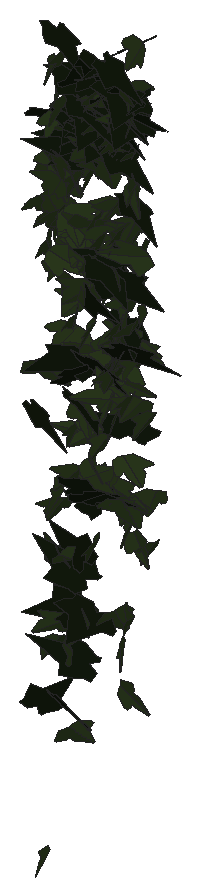
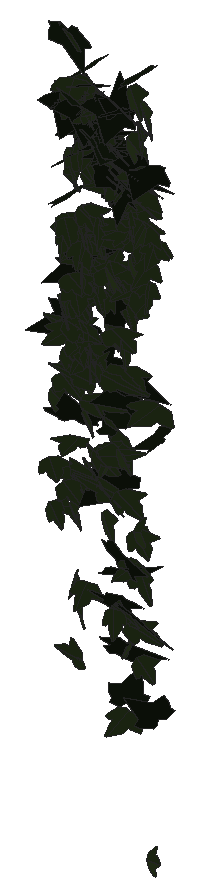
# SketchUp Ruby script. Lengths in millimetres.
U = 1.mm
M = Sketchup.active_model
def pt(a) = Geom::Point3d.new(a.map { |v| v * U })
def face(e, loops, mat)
  f = e.add_face(loops[0].map { |a| pt(a) })
  loops[1..].each { |l| e.add_face(l.map { |a| pt(a) }).erase! }
  f.material = f.back_material = mat if mat
  f
end
# faces: each face lists its corners as indices into pts; further lists are holes
def faces(e, pts, list, mat = nil) = list.each { |f| face(e, (f[0].is_a?(Array) ? f : [f]).map { |l| l.map { |i| pts[i] } }, mat) }
# xy, xz, yz: faces in a plane at the given z, y or x. An outline is a flat list of corners, or four numbers for a rectangle; further outlines are holes
def ring(l) = l.size == 4 ? [[l[0], l[1]], [l[2], l[1]], [l[2], l[3]], [l[0], l[3]]] : l.each_slice(2).to_a
def flat(e, list, mat, &to3) = list.each { |f| face(e, (f[0].is_a?(Array) ? f : [f]).map { |l| ring(l).map { |u, v| to3.(u, v) } }, mat) }
def xy(e, z, list, mat = nil) = flat(e, list, mat) { |x, y| [x, y, z] }
def xz(e, y, list, mat = nil) = flat(e, list, mat) { |x, z| [x, y, z] }
def yz(e, x, list, mat = nil) = flat(e, list, mat) { |y, z| [x, y, z] }
def lines(e, pts, list) = list.each { |a, b| e.add_line(pt(pts[a]), pt(pts[b])) }
# prism: a flat outline (further loops are holes) pulled along v
def prism(e, loops, v, mat = nil)
  f = face(e, loops, mat); d = Geom::Vector3d.new(v.map { |x| x * U })
  f.pushpull(f.normal.samedirection?(d) ? d.length : -d.length)
end
def box(e, o, s, mat = nil) = prism(e, [[o, [o[0] + s[0], o[1], o[2]], [o[0] + s[0], o[1] + s[1], o[2]], [o[0], o[1] + s[1], o[2]]]], [0, 0, s[2]], mat)
def at(x, y, z, deg = 0) = Geom::Transformation.translation(pt([x, y, z])) * Geom::Transformation.rotation(ORIGIN, Z_AXIS, deg.degrees)
def axes(o, x, y, z) = Geom::Transformation.new([*x, 0, *y, 0, *z, 0, *pt(o).to_a, 1])
def part(name) = M.definitions.add(name)
# library, detail: a bought-in or finely detailed component or shape, given as its bounding box
def library(name, o, s) = part(name).tap { |d| box(d.entities, o, s) }
def detail(e, o, s) = box(e.add_group.entities, o, s)
def put(e, d, t, mat = nil) = e.add_instance(d, t).tap { |i| i.material = mat if mat }
def group(e, t, mat = nil) = e.add_group.tap { |g| g.transformation = t; g.material = mat if mat }.entities
root = M.entities
M.materials.add("efeu1").color = [18, 25, 13]
M.materials.add("efeu2").color = [43, 57, 29]
c1 = part("ivyleaf_10")
p = [[0,12.8,-0.8],[-1.5,51.3,-10.9],[-4.9,51,-11.6],[-13.6,26.5,-7.3],[-13.2,15.9,-4.6],[-21.1,19.3,-7.2],
  [-29.5,16.3,-8.3],[-29.2,8.3,-6.2],[-19.7,-9.8,0.5],[-7.6,-13,4],[1,-12.2,5.8],[-0.4,51.1,-11.1],
  [-1.5,51.1,-10.9],[1,-12.4,5.9],[16.9,-12.4,3.5],[35.1,9.1,-5.1],[35,12.9,-6.1],[20.5,16.4,-4.9],
  [15.8,15,-3.8],[15.3,27.6,-7.1],[12.8,31.3,-7.8]]
faces(c1.entities,p,[[0,1,2,3,4,5,6,7,8,9,10],[11,12,0,13,14,15,16,17,18,19,20]],"efeu2")
c2 = part("ivyleaf_9")
p = [[39.1,54.8,31.7],[34.5,51.8,30.2],[-5.3,25.2,17.3],[-17.9,28.3,20.9],[-21.6,21.7,17],[-20.2,4.3,5.3],
  [-22.9,-0.3,2.5],[-17.1,-4,-0.6],[-2,-2.1,-1.2],[-0.7,-15.4,-10.1],[16.6,-22.3,-16.7],[21.1,-15.1,-12.5],
  [32.7,-10.7,-11],[46.1,-1.8,-6.6],[30.8,11.2,3.8]]
faces(c2.entities,p,[[0,1,2,3,4,5,6,7,8,9,10,11,12,13,14]],"efeu1")
put(root,c1,axes([1082.1,997.6,1167.9],[-0.50064,-0.61,-0.35285],[0.27301,0.3224,-0.66429],[1.31311,-0.2996,0.00358]))
put(root,c1,axes([1101.4,1010.7,594.9],[-0.91283,0.27362,0.57924],[-0.97949,0.2663,-0.55195],[-0.726,-0.70331,0.01636]))
put(root,c1,axes([1078.7,1010.7,105.8],[0.19332,-0.35249,0.55094],[0.37543,-0.51507,-0.36591],[1.18682,0.22035,0.02601]))
put(root,c1,axes([1074.1,1009.7,891.8],[-1.05756,-0.30294,-0.44533],[0.73832,0.21874,-0.63287],[0.71108,-0.67767,-0.0052]))
put(root,c1,axes([1088.7,1021.1,449.9],[-0.25395,-0.6181,0.25042],[-0.05666,-0.24961,-0.63195],[1.26798,-0.13495,0.02191]))
put(root,c1,axes([1084.8,1003.8,1095.4],[0.04007,-0.60352,-0.39627],[0.15482,0.3959,-0.59863],[1.36534,-0.02718,0.07951]))
put(root,c1,axes([1092.3,1026.2,670.5],[-0.45383,-0.63166,0.16282],[-0.10698,-0.15281,-0.67517],[1.23686,-0.24499,0.00134]))
put(root,c1,axes([1082.9,1012,1137.2],[-0.40105,-0.48424,-0.52608],[0.41583,0.47861,-0.52806],[1.29573,-0.30348,0.00664]))
put(root,c2,axes([1076.6,999.2,351.1],[-0.19601,-0.125,0.77139],[1.22033,0.43123,0.15549],[-0.85013,0.64784,0.04534]))
put(root,c2,axes([1089.8,1004.8,1306.5],[0.94112,0.57643,-0.03673],[-0.03109,-0.03438,-0.7594],[-1.09884,0.49466,-0.00998]))
put(root,c1,axes([1088.6,1027.2,680.6],[0.18777,-0.34057,0.59703],[0.34191,-0.56941,-0.3545],[1.26267,0.20483,0.00721]))
put(root,c1,axes([1088.2,1014.1,1202.2],[-1.29311,0.17274,-0.25591],[0.38946,-0.21125,-0.6859],[-0.44002,-0.69462,0.14496]))
put(root,c1,axes([1093.1,1017.7,1201.6],[-0.82238,0.6065,-0.06494],[-0.00615,-0.08186,-0.74301],[-1.16087,-0.42922,0.04994]))
put(root,c2,axes([1078,986.1,831.8],[0.78555,-0.62654,-0.12931],[-0.11182,0.11611,-0.75014],[1.21242,0.41666,0.0146]))
put(root,c1,axes([1094.3,1004.2,1165.7],[-0.99959,-0.46966,-0.21119],[0.33178,0.12169,-0.70416],[0.92221,-0.55285,0.02442]))
put(root,c1,axes([1100.8,1014.2,1059.6],[-0.24643,-0.28298,-0.65862],[-0.37765,-0.62898,0.30926],[-1.31099,0.23438,0.03472]))
put(root,c1,axes([1113,1005.1,495.6],[-0.47556,-0.35753,0.52872],[-0.54144,-0.44589,-0.43597],[1.0874,-0.37838,0.01416]))
put(root,c1,axes([1112.1,1004.2,1200.1],[-1.30805,-0.15889,0.23378],[-0.39038,-0.14256,-0.69991],[0.37015,-0.71183,0.08799]))
put(root,c1,axes([1106,991.6,1390.4],[0.42905,-0.74177,-0.16767],[-0.04749,0.16757,-0.77489],[1.44657,0.22551,0.02429]))
put(root,c1,axes([1107.2,998.6,1150.8],[-0.31003,-0.69789,-0.14303],[0.01023,0.14551,-0.71613],[1.35579,-0.16068,-0.0273]))
put(root,c1,axes([1104.8,1010.5,1294.6],[0.87098,0.52911,-0.30696],[-0.37355,-0.23608,-0.69955],[-1.10265,0.49792,-0.00548]))
put(root,c2,axes([1131.2,1007.8,520.9],[-1.29567,0.40892,0.16753],[-0.28984,0.07174,-0.79399],[-0.78952,-0.69742,0.01655]))
put(root,c1,axes([1108.5,1015.1,1138.7],[0.17279,-0.70124,0.16255],[0.06123,-0.15972,-0.707],[1.36861,0.09568,0.01111]))
put(root,c1,axes([1102.7,1008.5,1255.8],[-1.36787,-0.06482,-0.23032],[0.44252,-0.01725,-0.72073],[0.1074,-0.75453,0.03627]))
put(root,c1,axes([1110.5,988.8,1249.3],[-1.2264,0.40383,0.02809],[-0.04325,0.01664,-0.76047],[-0.76921,-0.64478,-0.00203]))
put(root,c1,axes([1108.2,1009.4,1232.4],[1.36759,0.22334,-0.06726],[-0.1882,0.0944,-0.74301],[-0.40205,0.71551,0.11902]))
put(root,c1,axes([1119.9,1026.3,729.2],[-0.43065,-0.60056,0.38096],[-0.23149,-0.36121,-0.64167],[1.33361,-0.25663,0.01164]))
put(root,c1,axes([1116.2,1024.3,953.1],[1.20348,0.14456,-0.26709],[-0.48948,-0.07321,-0.64853],[-0.30739,0.68252,-0.01299]))
put(root,c1,axes([1116,991.2,1356.8],[0.36278,-0.66633,-0.3782],[-0.04996,0.38382,-0.68946],[1.45733,0.17903,0.07051]))
put(root,c2,axes([1140.8,1008.7,1255.6],[-0.55107,0.56514,0.4192],[-0.59728,0.302,-0.6239],[-1.19859,-0.41032,0.11817]))
put(root,c2,axes([1133.9,1011.5,922.8],[0.0113,0.02878,-0.77488],[-0.45209,-0.73758,-0.02921],[-1.40481,0.2376,0.00317]))
put(root,c1,axes([1119.9,1002.8,1335.2],[0.15934,-0.74234,0.35722],[0.07303,-0.35515,-0.74704],[1.56618,0.09209,-0.00151]))
put(root,c1,axes([1123.1,1007.9,1212.6],[0.53883,-0.59272,-0.38248],[-0.12209,0.38879,-0.64999],[1.33698,0.27438,0.09479]))
put(root,c1,axes([1124.9,995.6,1416.9],[0.07108,-0.79445,-0.01493],[0.00122,0.01498,-0.79533],[1.51226,0.03733,0.00134]))
put(root,c1,axes([1124.2,1023.6,804.2],[0.09288,-0.67709,0.14502],[0.04312,-0.14374,-0.67874],[1.31715,0.05245,0.01199]))
put(root,c1,axes([1132.2,1028.4,1010.8],[-0.84414,-0.37253,0.40167],[-0.26402,-0.42359,-0.54605],[1.00865,-0.42265,0.19322]))
put(root,c2,axes([1147,1006.6,605.4],[-0.21405,0.22175,0.77835],[-0.63986,0.70202,-0.24858],[-1.40111,-0.35447,-0.00539]))
put(root,c1,axes([1127.5,1013.2,987.1],[0.03342,-0.64293,-0.28401],[0.01993,0.28431,-0.64295],[1.33754,0.01183,0.01668]))
put(root,c1,axes([1117.5,1004.4,602],[-0.46402,-0.34169,-0.54236],[0.58609,0.44648,-0.41972],[1.06998,-0.39274,-0.0053]))
put(root,c2,axes([1147.7,1006.4,577.8],[-1.15246,-0.54413,-0.08264],[-0.11643,-0.05556,0.8141],[-1.04097,0.60862,0.00043]))
put(root,c1,axes([1146.3,1022.8,927.1],[0.57425,0.17419,-0.66056],[-1.23973,-0.14423,-0.33557],[-0.39176,0.71174,0.09366]))
put(root,c1,axes([1142.3,1031.4,795.4],[0.18419,0.21341,0.70114],[-0.65067,-0.61242,0.23359],[1.23379,-0.35483,0.01852]))
put(root,c1,axes([1115.1,993.5,1086.7],[0.36131,0.51236,0.58931],[0.40782,0.54901,-0.54636],[-1.42915,0.2862,-0.00692]))
put(root,c2,axes([1155.2,1009.2,1288],[-1.20048,0.3657,0.23302],[-0.48153,0.02367,-0.72203],[-0.67024,-0.67202,0.10137]))
put(root,c2,axes([1137.8,1012.6,1255.1],[0.82971,0.02046,-0.62236],[-1.15513,0.18376,-0.41912],[0.26487,0.7373,0.12172]))
put(root,c1,axes([1135.4,1011.8,1253.1],[-0.79983,-0.62854,0.07317],[0.06392,-0.10987,-0.75089],[1.20261,-0.41219,0.08857]))
put(root,c2,axes([1160.9,998.9,447.2],[-0.93743,-0.24603,-0.52245],[-0.84954,-0.27346,0.54961],[-0.69731,0.66392,0.03277]))
put(root,c1,axes([1136.8,999.2,1046.3],[1.00577,-0.33956,-0.35804],[-0.31716,0.37098,-0.5978],[0.88396,0.51946,0.19289]))
put(root,c2,axes([1115.6,992.1,1449.5],[0.37601,-0.77601,-0.0574],[0.01079,0.06066,-0.80051],[1.4809,0.19659,0.02041]))
put(root,c1,axes([1130.2,1005.8,449.2],[-0.46563,0.54231,0.45521],[0.3612,-0.41377,0.59493],[1.29822,0.30963,-0.00226]))
put(root,c1,axes([1135.8,999.1,1281.7],[-1.43565,0.15028,-0.02924],[0.04257,-0.03726,-0.76848],[-0.28825,-0.75398,0.03215]))
put(root,c2,axes([1166.7,994.4,1268.9],[-1.03408,0.10343,0.57262],[-1.06439,0.12351,-0.55297],[-0.30579,-0.77965,-0.01164]))
put(root,c1,axes([1158.3,995.4,507.2],[0.00733,0.00014,0.69704],[-1.25102,0.23193,0.00359],[-0.4414,-0.65733,0.00141]))
put(root,c1,axes([1139,995.4,1229.7],[-0.48665,0.66394,0.23671],[-0.27228,0.19768,-0.70901],[-1.3136,-0.28695,0.05927]))
put(root,c1,axes([1133.3,1011.9,1255.7],[-0.34521,0.73538,-0.06968],[0.01283,-0.0701,-0.75735],[-1.40578,-0.18122,0.0102]))
put(root,c2,axes([1123.2,997.4,894.2],[0.72994,0.33289,0.62618],[0.8142,0.45917,-0.50613],[-1.07645,0.57303,0.04179]))
put(root,c2,axes([1156.5,998.9,1310],[-1.12871,0.48941,-0.02115],[0.03222,-0.01271,-0.76892],[-0.93175,-0.5933,-0.00097]))
put(root,c2,axes([1134.7,996.8,359.8],[1.02425,-0.55853,0.0638],[-0.08093,0.04763,0.77562],[-1.06685,-0.53985,0.00242]))
put(root,c1,axes([1140.1,1000.5,1283.3],[-1.22249,0.4254,0.00059],[0.00093,0.00181,-0.77043],[-0.80962,-0.64233,-0.00178]))
put(root,c2,axes([1155.5,1006.4,1273.8],[-1.25604,0.31647,-0.2085],[0.26414,-0.18779,-0.72433],[-0.67117,-0.66615,0.10514]))
put(root,c1,axes([1145.6,1003.9,1224.1],[0.05482,-0.7296,0.21948],[0.01824,-0.21927,-0.73017],[1.44992,0.03034,0.00089]))
put(root,c2,axes([1168.3,1000.5,1393.6],[-0.93418,0.51373,0.33176],[-0.47002,0.22266,-0.71017],[-1.06476,-0.54902,0.02242]))
put(root,c1,axes([1137.3,999.3,332.6],[-0.64056,-0.4779,-0.51375],[0.52987,0.43207,-0.58431],[1.22579,-0.43651,-0.01589]))
put(root,c2,axes([1154.3,1009.6,1280],[-0.05565,0.65607,-0.39234],[-0.03291,-0.3931,-0.65604],[-1.45449,-0.0162,0.02986]))
put(root,c1,axes([1145.8,1016.7,511.4],[-0.38398,-0.63444,-0.20102],[0.08355,0.19691,-0.66552],[1.26386,-0.20577,-0.01708]))
put(root,c1,axes([1152.5,1018.9,1104.1],[-0.92403,-0.39747,0.37014],[-0.22551,-0.40699,-0.59247],[1.00877,-0.45506,0.2066]))
put(root,c1,axes([1152.9,1027.7,802.1],[-0.33785,-0.27541,0.58765],[-0.18843,-0.59062,-0.30671],[1.2207,-0.16739,0.1153]))
put(root,c1,axes([1124.4,1006.3,1106.5],[-0.65872,-0.03458,-0.6433],[1.08099,-0.36099,-0.28618],[-0.57858,-0.63507,0.1977]))
put(root,c1,axes([1144.7,1025.7,1112.4],[0.3298,-0.69293,0.32663],[0.18468,-0.31234,-0.71407],[1.44621,0.1979,0.0167]))
put(root,c1,axes([1145.7,1010.7,1267.3],[-0.70095,0.66637,0.04571],[-0.08029,0.02889,-0.76103],[-1.26868,-0.37,0.02291]))
put(root,c2,axes([1164.6,1005,1320.4],[-0.52769,0.71307,-0.10855],[-0.09594,-0.13517,-0.75916],[-1.36939,-0.26531,0.09502]))
put(root,c1,axes([1142.2,1007.7,1281.6],[-1.29319,0.1576,-0.31858],[0.41449,-0.35857,-0.64189],[-0.53459,-0.65925,0.27296]))
put(root,c1,axes([1129,1015.3,1114.9],[1.0758,0.19179,0.44458],[0.77718,0.17836,-0.59614],[-0.49513,0.69667,0.03024]))
put(root,c1,axes([1165,1000.1,1050.9],[-0.85468,-0.51344,0.43661],[-0.56878,-0.31855,-0.682],[1.14972,-0.53928,-0.01283]))
put(root,c1,axes([1144.8,985.8,1163.2],[0.5917,0.72514,0.04616],[0.03517,0.0423,-0.78898],[-1.38243,0.31145,-0.00032]))
put(root,c1,axes([1138,1019,836.9],[1.04706,-0.26282,0.35768],[0.61688,-0.15127,-0.6097],[0.5771,0.63853,0.00278]))
put(root,c2,axes([1147.5,994.8,1377.7],[0.6766,0.42955,0.54046],[-0.72466,-0.38509,0.55653],[1.096,-0.51979,0.03432]))
put(root,c2,axes([1161.4,1003.3,1308.1],[-1.40464,-0.12735,-0.1659],[0.30445,0.04825,-0.74868],[0.25642,-0.75492,-0.01986]))
put(root,c2,axes([1136.3,1018.6,843.8],[-0.00618,-0.57717,0.50536],[0.40408,-0.48631,-0.55404],[1.40301,0.13752,0.1618]))
put(root,c1,axes([1155.8,1008.9,1109.9],[0.52952,0.69295,-0.00425],[0.00294,0.00396,0.74672],[1.31885,-0.27823,0.00004]))
put(root,c2,axes([1138.8,998.9,1385.4],[0.20867,-0.72856,-0.40087],[0.06409,0.4079,-0.73213],[1.58134,0.07961,0.08257]))
put(root,c2,axes([1158.5,1002.5,1381.7],[0.63521,0.69709,0.11537],[-0.02517,0.13373,-0.7698],[-1.34452,0.32684,0.06892]))
put(root,c2,axes([1184.6,1001.6,711.5],[-1.06906,0.25617,-0.54675],[-0.97424,0.19396,0.61679],[0.60938,0.7595,0.0269]))
put(root,c2,axes([1156.9,989.6,1324.3],[0.75277,0.5153,0.42065],[0.28957,0.40633,-0.64083],[-1.23243,0.41022,0.10636]))
put(root,c1,axes([1161.9,1005.7,1307.5],[-1.16127,0.45764,-0.12235],[0.1231,-0.11716,-0.76079],[-0.89313,-0.61119,0.05423]))
put(root,c1,axes([1165.1,1031.1,792.3],[-0.05732,-0.53512,0.43757],[0.1327,-0.4381,-0.53098],[1.30888,0.02098,0.073]))
put(root,c1,axes([1168.9,998.6,1351.2],[-0.32892,-0.71901,0.22616],[0.00062,-0.2321,-0.73765],[1.43453,-0.16476,0.05217]))
put(root,c2,axes([1172.2,1002.4,530.1],[-1.32188,-0.30587,-0.09091],[0.16152,0.03286,-0.75892],[0.58543,-0.69971,0.0041]))
put(root,c1,axes([1170.9,997.5,1108.7],[0.17809,-0.53219,-0.58167],[-0.14272,0.57709,-0.54006],[1.49366,0.11859,0.01775]))
put(root,c1,axes([1149.3,997.9,1250.9],[-0.09537,-0.0651,-0.78608],[1.03899,0.56567,-0.08165],[1.08355,-0.54814,0.0091]))
put(root,c1,axes([1186,1022.1,870.2],[-0.23437,0.00717,0.69853],[-0.80771,-0.56416,-0.06903],[1.05603,-0.42991,0.10223]))
put(root,c1,axes([1147.9,984.7,1169.5],[-0.5524,-0.21236,-0.73377],[1.22271,0.35679,-0.35738],[0.7865,-0.70382,0.04023]))
put(root,c1,axes([1167.7,1003.5,1238.9],[0.41381,-0.66895,0.25142],[0.13134,-0.24192,-0.70334],[1.35373,0.22796,-0.00861]))
put(root,c2,axes([1177.5,1006.7,1315.9],[0.3544,0.49207,0.5669],[-0.16004,0.59408,-0.48804],[-1.41969,0.05587,0.19653]))
put(root,c1,axes([1171.2,996.2,992.6],[0.34995,-0.68333,0.09055],[0.01631,-0.09144,-0.70747],[1.31178,0.18343,-0.01536]))
put(root,c1,axes([1165,1027.9,945.1],[0.04765,-0.46652,0.54693],[0.48166,-0.50651,-0.44363],[1.28058,0.20787,0.14651]))
put(root,c1,axes([1170.9,1002.5,767.1],[-0.67671,0.64282,0.07293],[-0.07444,0.0617,-0.73459],[-1.22901,-0.35768,0.00434]))
put(root,c2,axes([1165.9,1010,1308.2],[-0.45729,-0.71737,-0.11227],[0.02371,0.11417,-0.75615],[1.38171,-0.23938,-0.02418]))
put(root,c2,axes([1193,1008.5,1307.8],[-1.13869,0.46887,0.06436],[-0.10781,0.03205,-0.76008],[-0.89425,-0.6009,0.00968]))
put(root,c1,axes([1194.7,986.3,1282.1],[-1.04605,-0.20402,0.51943],[-0.92855,-0.17826,-0.58627],[0.51561,-0.73493,-0.00199]))
put(root,c2,axes([1172.8,1002.1,1327.7],[-0.61999,-0.66853,0.20551],[-0.16151,-0.18725,-0.74366],[1.32127,-0.33659,0.00553]))
put(root,c1,axes([1165.5,1005.9,1092.5],[1.24085,-0.31371,0.18344],[0.30324,-0.09186,-0.7234],[0.62161,0.67103,-0.01328]))
put(root,c1,axes([1178.1,999.5,1335.6],[0.79793,-0.58988,-0.4084],[-0.13168,0.43757,-0.70304],[1.3591,0.38871,0.17166]))
put(root,c2,axes([1146.6,1003.8,1036.1],[0.66531,-0.1483,-0.68391],[1.32447,-0.00675,0.35718],[-0.1401,-0.76804,0.12891]))
put(root,c2,axes([1145.1,990.7,723.5],[0.74503,-0.08579,0.64541],[1.20216,-0.13259,-0.40074],[0.30051,0.74311,0.00301]))
put(root,c1,axes([1178.9,996.6,1363.8],[0.23431,-0.7276,0.27853],[0.08952,-0.27453,-0.73794],[1.48006,0.13179,0.00054]))
put(root,c1,axes([1183.8,1006.9,1061.8],[0.60673,-0.46577,-0.481],[-0.24817,0.47934,-0.5506],[1.24989,0.32127,0.12417]))
put(root,c2,axes([1166.9,989.9,722.3],[1.1089,0.44586,0.21678],[0.31866,0.13789,-0.73363],[-0.8881,0.60619,0.00743]))
put(root,c1,axes([1152.6,1018.4,725.9],[0.19504,-0.06125,-0.70118],[1.31278,-0.13223,0.11236],[-0.26651,-0.69618,0.04035]))
put(root,c1,axes([1183.9,988.5,653.3],[0.18451,-0.71984,-0.06707],[-0.03093,0.06549,-0.7263],[1.37558,0.09803,-0.00733]))
put(root,c2,axes([1164.2,1009.7,1307.1],[0.46026,-0.72367,0.05841],[0.01837,-0.05835,-0.76295],[1.38165,0.24185,-0.00931]))
put(root,c2,axes([1161,1002.5,1347.6],[0.76251,-0.65964,0.09574],[0.1079,-0.07757,-0.77174],[1.26399,0.40456,0.00812]))
put(root,c1,axes([1182.8,1003.8,1172.7],[-0.04509,-0.674,-0.33665],[0.13008,0.3335,-0.67251],[1.42795,-0.05166,0.05063]))
put(root,c1,axes([1163.6,989.6,1148.9],[-0.55162,-0.40496,0.62058],[0.88042,0.42168,0.49122],[-1.10173,0.53973,0.08184]))
put(root,c1,axes([1186.4,998.8,1321.9],[-0.23016,-0.75719,-0.14488],[0.06042,0.14163,-0.76673],[1.46597,-0.12472,0.00886]))
put(root,c1,axes([1182.1,992.1,1107.2],[-0.28921,-0.60983,-0.38522],[0.28044,0.35913,-0.62665],[1.34385,-0.20619,0.04787]))
put(root,c2,axes([1168,989.8,1356.8],[0.09303,-0.73348,-0.24714],[0.17993,0.25143,-0.72753],[1.46204,0.01573,0.10526]))
put(root,c1,axes([1172,1022.1,733.9],[0.80041,-0.45932,-0.32451],[0.45003,-0.22324,0.62242],[-0.97113,-0.48202,0.02097]))
put(root,c2,axes([1172.2,990,940.3],[1.53332,-0.10434,-0.13006],[-0.24351,0.02467,-0.81235],[0.20349,0.81571,0.00793]))
put(root,c1,axes([1169.3,998.5,749.6],[0.96435,-0.23136,-0.42913],[0.76036,-0.15767,0.55673],[-0.53177,-0.64501,0.01783]))
put(root,c2,axes([1181.3,1007.6,1316.2],[-0.25176,-0.75721,0.00239],[0.0169,-0.00398,-0.76862],[1.44102,-0.13225,0.00943]))
put(root,c2,axes([1193.3,1006.3,1312.5],[-0.98608,-0.56351,0.03808],[-0.02358,-0.04033,-0.76529],[1.07466,-0.51795,0.01815]))
put(root,c1,axes([1186.2,1017,872.6],[0.77558,-0.56305,0.27012],[0.2578,-0.23517,-0.69456],[1.16024,0.42864,-0.02624]))
put(root,c1,axes([1194.3,995.3,930.2],[0.1047,-0.63551,-0.29193],[-0.0253,0.29183,-0.63779],[1.33077,0.05555,0.01084]))
put(root,c1,axes([1194.9,993.4,1148.7],[0.1302,-0.73655,-0.10429],[0.01867,0.10561,-0.73947],[1.41566,0.06635,0.01934]))
put(root,c1,axes([1195.1,995.8,1380.2],[0.48617,-0.75301,-0.0026],[0.02951,0.00801,-0.79497],[1.43284,0.25534,0.01726]))
put(root,c1,axes([1189.7,1028.7,844.3],[0.55764,-0.62395,0.29477],[0.27838,-0.25681,-0.68899],[1.28351,0.32679,0.02137]))
put(root,c1,axes([1200.1,1013.4,1191.6],[-0.5051,-0.58044,0.37251],[-0.07172,-0.38634,-0.62883],[1.31066,-0.24483,0.10915]))
put(root,c1,axes([1198.1,1005.6,937.5],[0.11891,-0.58588,-0.42335],[0.01654,0.4255,-0.58759],[1.37559,0.04553,0.04366]))
put(root,c1,axes([1201.6,1013.3,1192.8],[-0.39939,-0.68234,0.19235],[-0.05049,-0.1929,-0.71324],[1.3483,-0.20935,0.03027]))
put(root,c1,axes([1197.9,1008.8,947.1],[-0.39238,-0.56097,0.45342],[0.16602,-0.4875,-0.56348],[1.3627,-0.10214,0.19921]))
put(root,c1,axes([1201.4,999.4,1363],[-0.40177,-0.75667,0.00177],[0.00066,-0.00193,-0.78557],[1.4401,-0.2111,0.00085]))
put(root,c1,axes([1185.7,1016.3,951.6],[0.84484,-0.40526,0.40246],[0.5783,-0.26403,-0.60102],[0.92041,0.53788,0.00821]))
put(root,c2,axes([1219.2,1006.7,1101.1],[-0.2213,-0.01381,0.75707],[-1.32892,-0.29432,-0.11261],[0.55743,-0.70714,0.03209]))
put(root,c1,axes([1202.9,1007.8,1141.6],[0.48288,-0.6628,-0.221],[0.00883,0.23672,-0.7046],[1.32969,0.23912,0.08494]))
put(root,c1,axes([1205.5,997.7,1091.9],[0.95487,-0.40557,-0.37692],[-0.22473,0.41858,-0.60756],[1.02951,0.46753,0.21697]))
put(root,c1,axes([1204.3,997.1,1366.7],[-0.83728,0.61897,0.18759],[-0.22286,0.14689,-0.75932],[-1.2106,-0.45514,0.01004]))
put(root,c1,axes([1204.7,991.6,1263.3],[-1.26281,-0.36756,-0.08633],[0.13385,0.05119,-0.75845],[0.706,-0.66715,-0.01063]))
put(root,c1,axes([1209.3,1012.8,1091.9],[0.20705,-0.59833,-0.40876],[0.01763,0.41446,-0.6042],[1.379,0.08454,0.0691]))
put(root,c1,axes([1219.9,1020.8,992.4],[-0.45233,-0.45278,0.56381],[-0.44312,-0.51396,-0.51089],[1.30294,-0.33198,0.02198]))
put(root,c1,axes([1205.2,1010.9,536.8],[-0.55046,-0.57839,-0.34318],[0.33386,0.29575,-0.64631],[1.23567,-0.33757,0.02175]))
put(root,c1,axes([1204,996.2,1365.2],[1.16896,0.48386,0.06294],[-0.16257,0.20625,-0.752],[-0.9143,0.58196,0.21418]))
put(root,c1,axes([1212.5,1012.7,934.1],[1.09801,0.31971,-0.32961],[-0.53082,-0.17649,-0.65937],[-0.69426,0.64058,-0.01716]))
put(root,c1,axes([1210.3,1005.5,1304],[-0.36562,-0.69056,-0.27825],[0.17607,0.26299,-0.71657],[1.40596,-0.21251,0.01738]))
put(root,c1,axes([1213.8,993.6,933],[-0.25046,-0.69862,0.05535],[-0.02555,-0.0538,-0.7109],[1.33353,-0.13224,-0.00322]))
put(root,c2,axes([1213.7,1001.3,1363.8],[0.58492,0.71573,-0.08509],[-0.04658,-0.08209,-0.77886],[-1.37097,0.30815,-0.00984]))
put(root,c1,axes([1208.2,1016.1,1129.4],[-0.55833,-0.67342,-0.10135],[0.34801,0.02841,-0.71804],[1.24849,-0.30907,0.15482]))
put(root,c2,axes([1202.5,999.4,1354.8],[1.16942,0.27668,0.39341],[-0.67301,-0.17274,0.67379],[0.62045,-0.70886,-0.01063]))
put(root,c1,axes([1213.3,1022.4,1033.1],[-0.27194,-0.64037,0.27812],[0.06283,-0.28977,-0.65022],[1.32726,-0.11749,0.08776]))
put(root,c1,axes([1207,1010.3,941.7],[-0.43991,-0.49201,-0.45452],[0.40204,0.40274,-0.54339],[1.20976,-0.31276,0.01531]))
put(root,c1,axes([1216.1,1019.6,961.5],[-0.49491,-0.62676,0.10728],[-0.05481,-0.10417,-0.67843],[1.20895,-0.2613,0.01316]))
put(root,c1,axes([1208.1,1002.7,1352.7],[-0.11096,0.73394,0.26021],[-0.05261,0.25882,-0.73622],[-1.48109,-0.06418,0.00666]))
put(root,c1,axes([1216.3,1007.5,1282.2],[-0.35414,-0.71305,0.19459],[-0.00592,-0.19991,-0.7355],[1.40669,-0.18035,0.04589]))
put(root,c2,axes([1198.6,992.2,1104.7],[0.11536,-0.74439,-0.2178],[0.04171,0.22002,-0.74588],[1.47554,0.05198,0.03811]))
put(root,c1,axes([1220.4,1023.2,1073],[-0.70768,-0.48015,0.37583],[-0.18406,-0.38819,-0.59162],[1.14578,-0.35891,0.13709]))
put(root,c1,axes([1217.3,1020.5,1053.3],[-0.68298,-0.62768,-0.01691],[-0.00907,0.0222,-0.72286],[1.195,-0.35857,-0.01516]))
put(root,c2,axes([1193.9,997.3,1350.2],[1.43343,-0.2063,-0.02432],[-0.04197,0.01157,-0.78089],[0.39311,0.75347,0.00533]))
put(root,c1,axes([1218.8,995.2,1308.7],[-0.04216,-0.75954,-0.15927],[0.07604,0.15801,-0.75907],[1.47503,-0.02985,0.03458]))
put(root,c1,axes([1217.2,1025.3,674.8],[0.42311,-0.61813,0.11505],[0.09865,-0.1036,-0.65676],[1.19256,0.22788,0.01351]))
put(root,c1,axes([1222.8,990.5,1372.1],[-0.80841,-0.67234,-0.00008],[0.01731,-0.00565,-0.7952],[1.27947,-0.42473,0.01071]))
put(root,c1,axes([1213.1,1000.7,1361.2],[0.56546,-0.59237,0.41737],[0.35252,-0.37403,-0.6627],[1.33333,0.35011,-0.0018]))
put(root,c1,axes([1223.5,991.5,1375.6],[1.11091,-0.47287,-0.23227],[-0.27696,0.18846,-0.74938],[0.96366,0.59929,0.05239]))
put(root,c1,axes([1222.6,998.9,1163.1],[0.11494,-0.70294,-0.22829],[-0.00996,0.22864,-0.7054],[1.40659,0.05906,0.01366]))
put(root,c1,axes([1220.3,990.9,1396.4],[-1.09316,0.53944,-0.02356],[0.0313,-0.0169,-0.78798],[-1.02716,-0.57462,0.00106]))
put(root,c1,axes([1228.6,1025.5,710.5],[-0.49392,-0.53289,0.29073],[-0.11514,-0.2919,-0.58905],[1.14957,-0.2582,0.06591]))
put(root,c1,axes([1225.4,1000.7,972.9],[0.46716,-0.75777,-0.06924],[-0.04035,0.06591,-0.79653],[1.44763,0.24637,0.00014]))
put(root,c1,axes([1226.7,986.9,1018.6],[0.11181,-0.71034,-0.13607],[-0.02285,0.13554,-0.71276],[1.37631,0.05996,-0.00078]))
put(root,c2,axes([1223.4,1017.5,829.6],[-1.14455,-0.06605,0.45913],[0.87753,-0.00307,0.6035],[-0.09636,0.7566,0.04253]))
put(root,c1,axes([1200.6,1014.6,735],[-0.33882,0.04055,-0.73109],[1.15264,-0.4147,-0.17048],[-0.78319,-0.62786,0.06538]))
put(root,c1,axes([1231,1016.3,1169.9],[-0.7641,-0.60587,0.15225],[-0.05335,-0.16333,-0.72387],[1.18774,-0.3971,0.06543]))
put(root,c1,axes([1197.1,1018.7,904.3],[-0.12968,-0.01687,0.7537],[1.42005,0.10671,0.06984],[-0.20517,0.74921,0.00703]))
put(root,c1,axes([1215.6,1010.5,489.2],[0.35032,-0.39832,0.53365],[0.60212,-0.43488,-0.43372],[1.1152,0.35992,0.06654]))
put(root,c1,axes([1215.5,1013.8,1120.3],[-1.10488,0.28027,-0.33803],[0.57325,-0.15358,-0.64462],[-0.60812,-0.65399,0.00652]))
put(root,c1,axes([1230.2,1013.3,1281.8],[-0.09997,-0.73593,-0.17359],[-0.00314,0.17412,-0.73768],[1.43906,-0.05074,-0.01367]))
put(root,c1,axes([1228.5,1026.6,943.1],[-0.08774,-0.61074,0.33039],[0.08539,-0.33304,-0.60939],[1.31878,-0.01907,0.06144]))
put(root,c1,axes([1222.1,1001.5,1025.4],[0.81648,-0.54847,0.24214],[0.28722,-0.18937,-0.69632],[1.10431,0.45477,0.00208]))
put(root,c2,axes([1211.7,982.1,1432.9],[0.69941,-0.61019,-0.37263],[-0.17913,0.37404,-0.70532],[1.3489,0.36606,0.09954]))
put(root,c1,axes([1231.7,1023.4,1164.8],[-0.42469,-0.69595,-0.00701],[0.03447,0.00155,-0.73066],[1.32416,-0.22325,0.01677]))
put(root,c1,axes([1232.7,991.6,1367.6],[-0.89774,0.58066,0.2194],[-0.3016,0.15377,-0.74769],[-1.14222,-0.49698,0.02499]))
put(root,c1,axes([1226.1,1003.3,722.1],[-1.24788,-0.31948,-0.21323],[0.37933,0.07762,-0.72917],[0.6249,-0.68509,0.01682]))
put(root,c1,axes([1230.4,1001.7,540.7],[0.16218,-0.31214,-0.62246],[0.05804,0.62817,-0.31084],[1.324,0.0107,0.08987]))
put(root,c2,axes([1210.4,995.7,1371.2],[0.69044,-0.69622,-0.03167],[0.09893,0.06264,-0.78148],[1.32272,0.35873,0.07498]))
put(root,c2,axes([1213.6,995.9,1084.1],[-0.09543,-0.18056,-0.77806],[0.51477,0.72969,-0.18677],[1.43034,-0.27466,0.0153]))
put(root,c2,axes([1216.9,997.3,1287.4],[0.46321,-0.61698,-0.40134],[-0.02419,0.41912,-0.65203],[1.40059,0.21129,0.12147]))
put(root,c1,axes([1237.9,990.8,1353.3],[-0.79661,-0.6469,0.12752],[0.08608,-0.17886,-0.75888],[1.25191,-0.39933,0.13333]))
put(root,c2,axes([1224.1,1016.7,1011.4],[-0.06884,-0.73349,0.24261],[-0.03109,-0.2421,-0.73436],[1.47002,-0.03947,-0.00417]))
put(root,c2,axes([1255.4,999,1383.5],[-0.98591,0.58635,-0.0881],[-0.09559,-0.15996,-0.76929],[-1.12441,-0.50053,0.14264]))
put(root,c1,axes([1244.1,1011.6,887.1],[-0.70473,-0.49175,0.32008],[-0.24664,-0.3006,-0.61174],[1.08912,-0.38627,0.06858]))
put(root,c1,axes([1225,1010.1,786.7],[0.6729,0.54241,0.22348],[0.23169,0.18741,-0.64746],[-1.09219,0.37393,0.00034]))
put(root,c2,axes([1211.8,1007.8,1330.2],[0.30604,-0.07307,-0.74769],[1.38392,-0.17697,0.17368],[-0.35922,-0.74403,0.03212]))
put(root,c1,axes([1239.5,997.4,900.5],[0.07058,-0.698,0.02112],[0.00729,-0.02095,-0.69898],[1.32902,0.03718,0.00271]))
put(root,c1,axes([1237.1,1003.5,1397.3],[-0.93836,-0.57297,-0.1927],[0.31054,0.1133,-0.75436],[1.10779,-0.5171,0.04824]))
put(root,c1,axes([1260.5,992.1,1137.9],[0.55222,0.00478,-0.68948],[-1.30894,-0.05107,-0.28978],[-0.09311,0.7463,-0.01541]))
put(root,c1,axes([1241.5,998.9,1015.2],[-0.10798,-0.73413,-0.01355],[0.00317,0.01347,-0.73632],[1.39744,-0.05676,0.00063]))
put(root,c2,axes([1236.4,997.8,1391],[-0.80132,-0.66146,0.09181],[0.05109,-0.12521,-0.779],[1.26994,-0.41234,0.08927]))
put(root,c1,axes([1244.3,1020.4,1023.5],[0.42182,-0.67623,-0.20192],[-0.08835,0.19722,-0.71143],[1.34024,0.22583,0.01665]))
put(root,c1,axes([1217.1,1015.1,413.6],[0.21185,-0.06283,0.68473],[1.23858,-0.2143,-0.12546],[0.42247,0.65978,0.02446]))
put(root,c2,axes([1243,996.5,1358.8],[-0.87923,-0.63034,0.04306],[-0.02719,-0.0429,-0.78138],[1.20215,-0.46199,0.01382]))
put(root,c2,axes([1256.6,989.6,1475.9],[-0.07924,0.79987,0.00752],[-0.08034,0.00532,-0.79986],[-1.52026,-0.04197,0.04188]))
put(root,c2,axes([1239.9,992.3,1357.1],[1.27625,0.3296,-0.23157],[-0.39128,-0.10669,-0.74719],[-0.65927,0.70137,-0.00483]))
put(root,c1,axes([1217.3,1014.4,983.2],[-0.17258,0.0637,-0.75894],[1.29198,-0.33974,-0.10962],[-0.65714,-0.68468,-0.01622]))
put(root,c1,axes([1248.1,1011.4,1136.5],[-0.14476,-0.67093,-0.29739],[0.14179,0.29038,-0.67417],[1.38952,-0.09953,0.03781]))
put(root,c1,axes([1251.1,983.1,1362.8],[0.5279,-0.64336,-0.34995],[-0.09741,0.35626,-0.69553],[1.39045,0.26922,0.08413]))
put(root,c1,axes([1238.7,1012.2,973.2],[-0.82619,-0.28898,-0.47445],[0.73719,0.27417,-0.52139],[0.75788,-0.5817,-0.01005]))
put(root,c1,axes([1254.1,984.6,1251.6],[0.43512,-0.59011,-0.41865],[-0.14812,0.41645,-0.62951],[1.36904,0.23261,0.06495]))
put(root,c1,axes([1252.2,1024.3,862.4],[-0.01973,-0.6171,0.38591],[0.05546,-0.38599,-0.61645],[1.3841,0.00667,0.0302]))
put(root,c2,axes([1235.4,1008.8,1209.1],[0.37747,-0.72895,-0.0819],[-0.02347,0.08151,-0.75539],[1.39586,0.19849,0.00945]))
put(root,c2,axes([1229.9,984.9,979.7],[1.42484,0.1371,0.35798],[0.6638,0.0823,-0.76093],[-0.30273,0.82575,0.0164]))
put(root,c1,axes([1237.4,1011.7,667.3],[0.74841,-0.22962,0.57025],[0.97388,-0.2529,-0.4547],[0.64841,0.64488,0.02473]))
put(root,c1,axes([1260.4,1021.1,660.7],[-0.09937,-0.63909,0.12976],[-0.00783,-0.12985,-0.64119],[1.24112,-0.05199,0.00635]))
put(root,c1,axes([1258.9,990.9,1472.6],[0.97266,-0.61334,-0.0575],[-0.06228,0.04758,-0.79834],[1.17078,0.51208,0.0053]))
put(root,c1,axes([1261.2,1025,740.8],[-0.58769,-0.54295,0.15479],[0.0714,-0.19577,-0.61186],[1.07215,-0.28458,0.12559]))
put(root,c1,axes([1242.1,999.6,1236.9],[0.63725,-0.27376,0.646],[0.93026,-0.42248,-0.43239],[0.95793,0.59239,-0.00984]))
